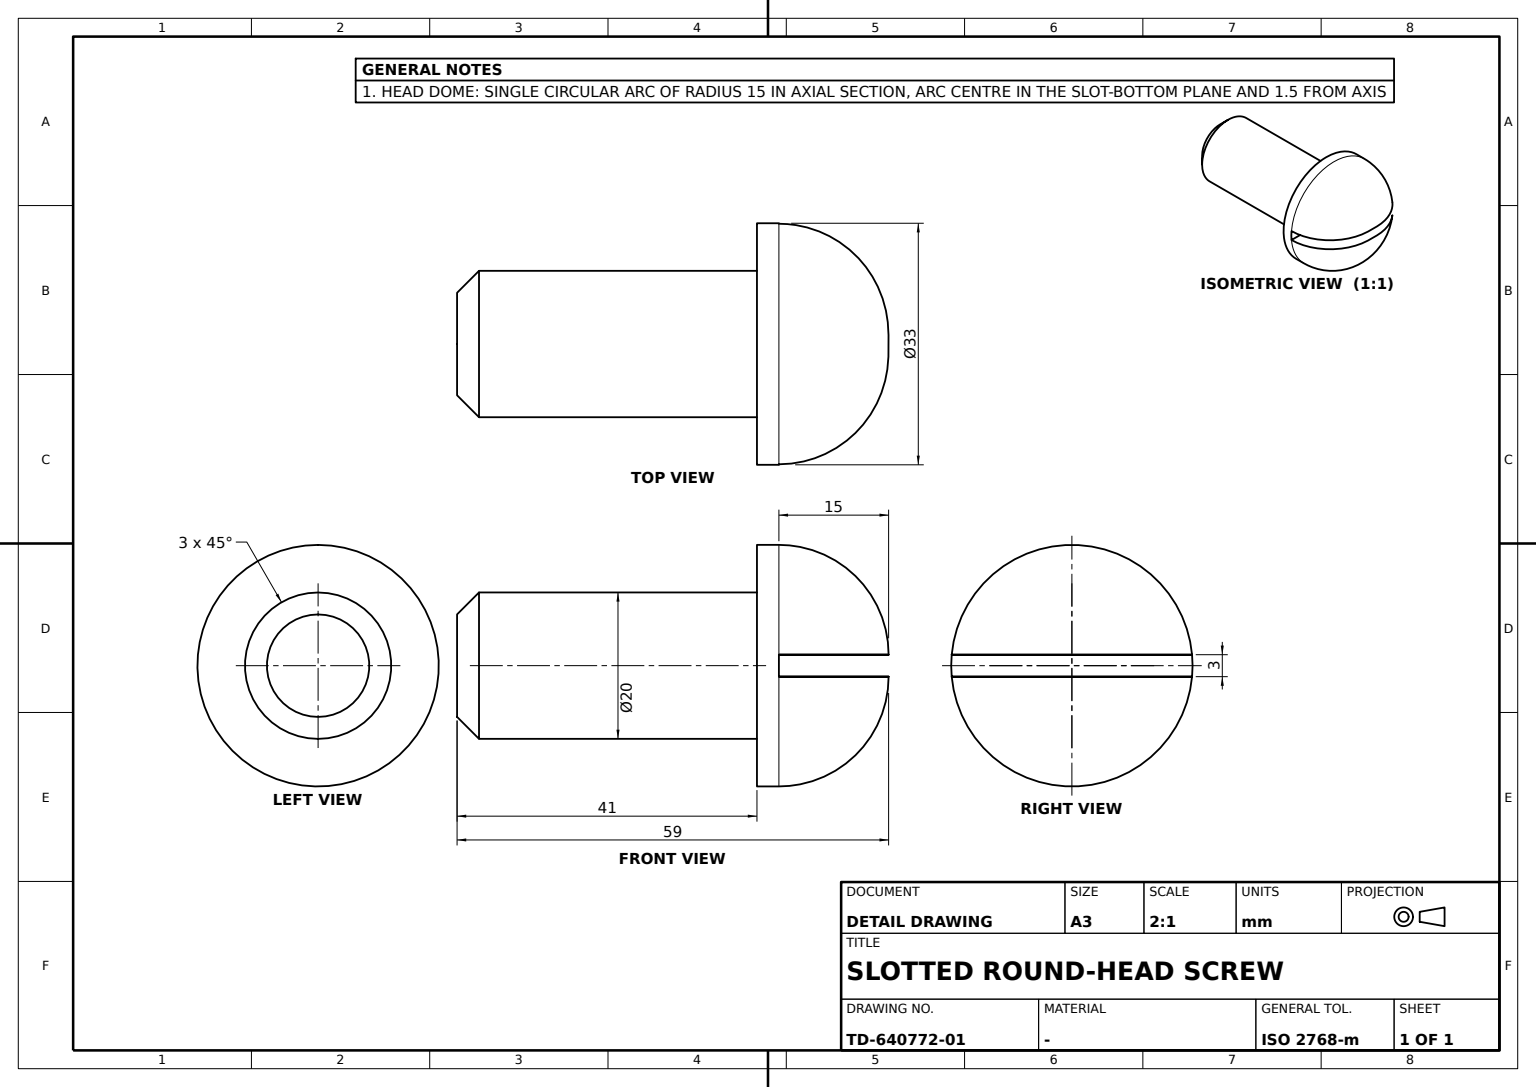
ISO-10303-21;
HEADER;
FILE_DESCRIPTION((''),'2;1');
FILE_NAME('','',(''),(''),'','','');
FILE_SCHEMA(('AUTOMOTIVE_DESIGN'));
ENDSEC;
DATA;
#1=APPLICATION_CONTEXT('');
#2=PRODUCT_CONTEXT('',#1,'mechanical');
#3=PRODUCT('','','',(#2));
#4=PRODUCT_DEFINITION_FORMATION('','',#3);
#5=PRODUCT_DEFINITION_CONTEXT('',#1,'design');
#6=PRODUCT_DEFINITION('','',#4,#5);
#7=PRODUCT_DEFINITION_SHAPE('','',#6);
#8=(LENGTH_UNIT()NAMED_UNIT(*)SI_UNIT(.MILLI.,.METRE.));
#9=(NAMED_UNIT(*)PLANE_ANGLE_UNIT()SI_UNIT($,.RADIAN.));
#10=(NAMED_UNIT(*)SI_UNIT($,.STERADIAN.)SOLID_ANGLE_UNIT());
#11=UNCERTAINTY_MEASURE_WITH_UNIT(LENGTH_MEASURE(0.005),#8,'distance_accuracy_value','');
#12=(GEOMETRIC_REPRESENTATION_CONTEXT(3)GLOBAL_UNCERTAINTY_ASSIGNED_CONTEXT((#11))GLOBAL_UNIT_ASSIGNED_CONTEXT((#8,#9,#10))REPRESENTATION_CONTEXT('',''));
#13=CARTESIAN_POINT('',(-56.,0.,-10.));
#14=VERTEX_POINT('',#13);
#15=CARTESIAN_POINT('',(-56.,0.,0.));
#16=DIRECTION('',(1.,0.,0.));
#17=DIRECTION('',(0.,0.,-1.));
#18=AXIS2_PLACEMENT_3D('',#15,#16,#17);
#19=CIRCLE('',#18,10.);
#20=EDGE_CURVE('',#14,#14,#19,.F.);
#21=ORIENTED_EDGE('',*,*,#20,.F.);
#22=EDGE_LOOP('',(#21));
#23=FACE_BOUND('',#22,.T.);
#24=CARTESIAN_POINT('',(-18.,0.,10.));
#25=VERTEX_POINT('',#24);
#26=CARTESIAN_POINT('',(-18.,0.,0.));
#27=DIRECTION('',(-1.,0.,0.));
#28=DIRECTION('',(0.,0.,1.));
#29=AXIS2_PLACEMENT_3D('',#26,#27,#28);
#30=CIRCLE('',#29,10.);
#31=EDGE_CURVE('',#25,#25,#30,.T.);
#32=ORIENTED_EDGE('',*,*,#31,.T.);
#33=EDGE_LOOP('',(#32));
#34=FACE_BOUND('',#33,.T.);
#35=CARTESIAN_POINT('',(-29.5,0.,0.));
#36=DIRECTION('',(0.,1.,0.));
#37=AXIS2_PLACEMENT_3D('',#35,#27,#36);
#38=CYLINDRICAL_SURFACE('',#37,10.);
#39=ADVANCED_FACE('',(#23,#34),#38,.T.);
#40=CARTESIAN_POINT('',(-15.,-16.431677,-1.5));
#41=VERTEX_POINT('',#40);
#42=CARTESIAN_POINT('',(-15.,16.431677,-1.5));
#43=VERTEX_POINT('',#42);
#44=CARTESIAN_POINT('',(-12.903045,-16.431677,-1.5));
#45=CARTESIAN_POINT('',(-8.772785,-15.550585,-1.5));
#46=CARTESIAN_POINT('',(-3.603958,-11.819536,-1.5));
#47=CARTESIAN_POINT('',(-0.941633,-7.253015,-1.5));
#48=CARTESIAN_POINT('',(-0.02238,-3.154463,-1.5));
#49=CARTESIAN_POINT('',(0.010788,-0.0197,-1.5));
#50=CARTESIAN_POINT('',(-0.020773,3.114717,-1.5));
#51=CARTESIAN_POINT('',(-0.906293,7.157145,-1.5));
#52=CARTESIAN_POINT('',(-3.570782,11.795182,-1.5));
#53=CARTESIAN_POINT('',(-8.743115,15.539047,-1.5));
#54=CARTESIAN_POINT('',(-12.897308,16.431677,-1.5));
#55=B_SPLINE_CURVE_WITH_KNOTS('',3,(#40,#44,#45,#46,#47,#48,#49,#50,#51,#52,#53,#54,#42),.UNSPECIFIED.,.F.,.F.,(4,1,1,1,1,1,1,1,1,1,4),(0.,0.006201557,0.012403114,0.018604671,0.021705449,0.024806228,0.027907006,0.031007785,0.037209342,0.043410898,0.049612455),.UNSPECIFIED.);
#56=EDGE_CURVE('',#41,#43,#55,.T.);
#57=ORIENTED_EDGE('',*,*,#56,.T.);
#58=CARTESIAN_POINT('',(-15.,16.5,-1.5));
#59=DIRECTION('',(0.,-1.,0.));
#60=VECTOR('',#59,1000.);
#61=LINE('',#58,#60);
#62=EDGE_CURVE('',#43,#41,#61,.T.);
#63=ORIENTED_EDGE('',*,*,#62,.T.);
#64=EDGE_LOOP('',(#57,#63));
#65=FACE_BOUND('',#64,.T.);
#66=CARTESIAN_POINT('',(0.,16.5,-1.5));
#67=AXIS2_PLACEMENT_3D('',#66,#17,#59);
#68=PLANE('',#67);
#69=ADVANCED_FACE('',(#65),#68,.F.);
#70=CARTESIAN_POINT('',(-15.,-16.431677,1.5));
#71=VERTEX_POINT('',#70);
#72=CARTESIAN_POINT('',(-15.,16.431677,1.5));
#73=VERTEX_POINT('',#72);
#74=CARTESIAN_POINT('',(-15.,-16.5,1.5));
#75=VECTOR('',#36,1000.);
#76=LINE('',#74,#75);
#77=EDGE_CURVE('',#71,#73,#76,.T.);
#78=ORIENTED_EDGE('',*,*,#77,.F.);
#79=CARTESIAN_POINT('',(-15.,0.,0.));
#80=AXIS2_PLACEMENT_3D('',#79,#16,#17);
#81=CIRCLE('',#80,16.5);
#82=EDGE_CURVE('',#71,#41,#81,.T.);
#83=ORIENTED_EDGE('',*,*,#82,.T.);
#84=ORIENTED_EDGE('',*,*,#62,.F.);
#85=EDGE_CURVE('',#43,#73,#81,.T.);
#86=ORIENTED_EDGE('',*,*,#85,.T.);
#87=EDGE_LOOP('',(#78,#83,#84,#86));
#88=FACE_BOUND('',#87,.T.);
#89=AXIS2_PLACEMENT_3D('',#79,#16,#36);
#90=PLANE('',#89);
#91=ADVANCED_FACE('',(#88),#90,.T.);
#92=CARTESIAN_POINT('',(-12.896233,-16.431677,1.5));
#93=CARTESIAN_POINT('',(-8.752476,-15.54483,1.5));
#94=CARTESIAN_POINT('',(-3.574351,-11.790403,1.5));
#95=CARTESIAN_POINT('',(-0.917122,-7.200652,1.5));
#96=CARTESIAN_POINT('',(-0.015222,-3.081954,1.5));
#97=CARTESIAN_POINT('',(0.010861,0.046159,1.5));
#98=CARTESIAN_POINT('',(-0.028223,3.200533,1.5));
#99=CARTESIAN_POINT('',(-0.943132,7.240634,1.5));
#100=CARTESIAN_POINT('',(-3.601842,11.822174,1.5));
#101=CARTESIAN_POINT('',(-8.775132,15.551126,1.5));
#102=CARTESIAN_POINT('',(-12.905796,16.431677,1.5));
#103=B_SPLINE_CURVE_WITH_KNOTS('',3,(#70,#92,#93,#94,#95,#96,#97,#98,#99,#100,#101,#102,#72),.UNSPECIFIED.,.F.,.F.,(4,1,1,1,1,1,1,1,1,1,4),(0.,0.006221705,0.012443411,0.018665116,0.021775968,0.024886821,0.027997674,0.031108526,0.037330232,0.043551937,0.049773642),.UNSPECIFIED.);
#104=EDGE_CURVE('',#71,#73,#103,.T.);
#105=ORIENTED_EDGE('',*,*,#104,.T.);
#106=AXIS2_PLACEMENT_3D('',#79,#27,#28);
#107=CIRCLE('',#106,16.5);
#108=EDGE_CURVE('',#71,#73,#107,.T.);
#109=ORIENTED_EDGE('',*,*,#108,.F.);
#110=EDGE_LOOP('',(#105,#109));
#111=FACE_BOUND('',#110,.T.);
#112=AXIS2_PLACEMENT_3D('',#79,#27,#36);
#113=DEGENERATE_TOROIDAL_SURFACE('',#112,1.5,15.,.T.);
#114=ADVANCED_FACE('',(#111),#113,.T.);
#115=ORIENTED_EDGE('',*,*,#104,.F.);
#116=ORIENTED_EDGE('',*,*,#77,.T.);
#117=EDGE_LOOP('',(#115,#116));
#118=FACE_BOUND('',#117,.T.);
#119=CARTESIAN_POINT('',(0.,-16.5,1.5));
#120=AXIS2_PLACEMENT_3D('',#119,#28,#36);
#121=PLANE('',#120);
#122=ADVANCED_FACE('',(#118),#121,.F.);
#123=ORIENTED_EDGE('',*,*,#31,.F.);
#124=EDGE_LOOP('',(#123));
#125=FACE_BOUND('',#124,.T.);
#126=CARTESIAN_POINT('',(-18.,0.,16.5));
#127=VERTEX_POINT('',#126);
#128=CIRCLE('',#29,16.5);
#129=EDGE_CURVE('',#127,#127,#128,.T.);
#130=ORIENTED_EDGE('',*,*,#129,.T.);
#131=EDGE_LOOP('',(#130));
#132=FACE_BOUND('',#131,.T.);
#133=AXIS2_PLACEMENT_3D('',#126,#27,#36);
#134=PLANE('',#133);
#135=ADVANCED_FACE('',(#125,#132),#134,.T.);
#136=CARTESIAN_POINT('',(-59.,0.,7.));
#137=VERTEX_POINT('',#136);
#138=CARTESIAN_POINT('',(-59.,0.,0.));
#139=AXIS2_PLACEMENT_3D('',#138,#27,#28);
#140=CIRCLE('',#139,7.);
#141=EDGE_CURVE('',#137,#137,#140,.T.);
#142=ORIENTED_EDGE('',*,*,#141,.F.);
#143=EDGE_LOOP('',(#142));
#144=FACE_BOUND('',#143,.T.);
#145=ORIENTED_EDGE('',*,*,#20,.T.);
#146=EDGE_LOOP('',(#145));
#147=FACE_BOUND('',#146,.T.);
#148=CARTESIAN_POINT('',(-66.,0.,0.));
#149=DIRECTION('',(0.,0.140359991,0.990100537));
#150=AXIS2_PLACEMENT_3D('',#148,#16,#149);
#151=CONICAL_SURFACE('',#150,0.,0.785398163);
#152=ADVANCED_FACE('',(#144,#147),#151,.T.);
#153=ORIENTED_EDGE('',*,*,#82,.F.);
#154=ORIENTED_EDGE('',*,*,#108,.T.);
#155=ORIENTED_EDGE('',*,*,#85,.F.);
#156=EDGE_CURVE('',#43,#41,#107,.T.);
#157=ORIENTED_EDGE('',*,*,#156,.T.);
#158=EDGE_LOOP('',(#153,#154,#155,#157));
#159=FACE_BOUND('',#158,.T.);
#160=ORIENTED_EDGE('',*,*,#129,.F.);
#161=EDGE_LOOP('',(#160));
#162=FACE_BOUND('',#161,.T.);
#163=CYLINDRICAL_SURFACE('',#37,16.5);
#164=ADVANCED_FACE('',(#159,#162),#163,.T.);
#165=ORIENTED_EDGE('',*,*,#56,.F.);
#166=ORIENTED_EDGE('',*,*,#156,.F.);
#167=EDGE_LOOP('',(#165,#166));
#168=FACE_BOUND('',#167,.T.);
#169=ADVANCED_FACE('',(#168),#113,.T.);
#170=ORIENTED_EDGE('',*,*,#141,.T.);
#171=EDGE_LOOP('',(#170));
#172=FACE_BOUND('',#171,.T.);
#173=CARTESIAN_POINT('',(-59.,0.,10.));
#174=AXIS2_PLACEMENT_3D('',#173,#27,#36);
#175=PLANE('',#174);
#176=ADVANCED_FACE('',(#172),#175,.T.);
#177=CLOSED_SHELL('',(#39,#69,#91,#114,#122,#135,#152,#164,#169,#176));
#178=MANIFOLD_SOLID_BREP('',#177);
#179=ADVANCED_BREP_SHAPE_REPRESENTATION('',(#178),#12);
#180=SHAPE_DEFINITION_REPRESENTATION(#7,#179);
ENDSEC;
END-ISO-10303-21;
